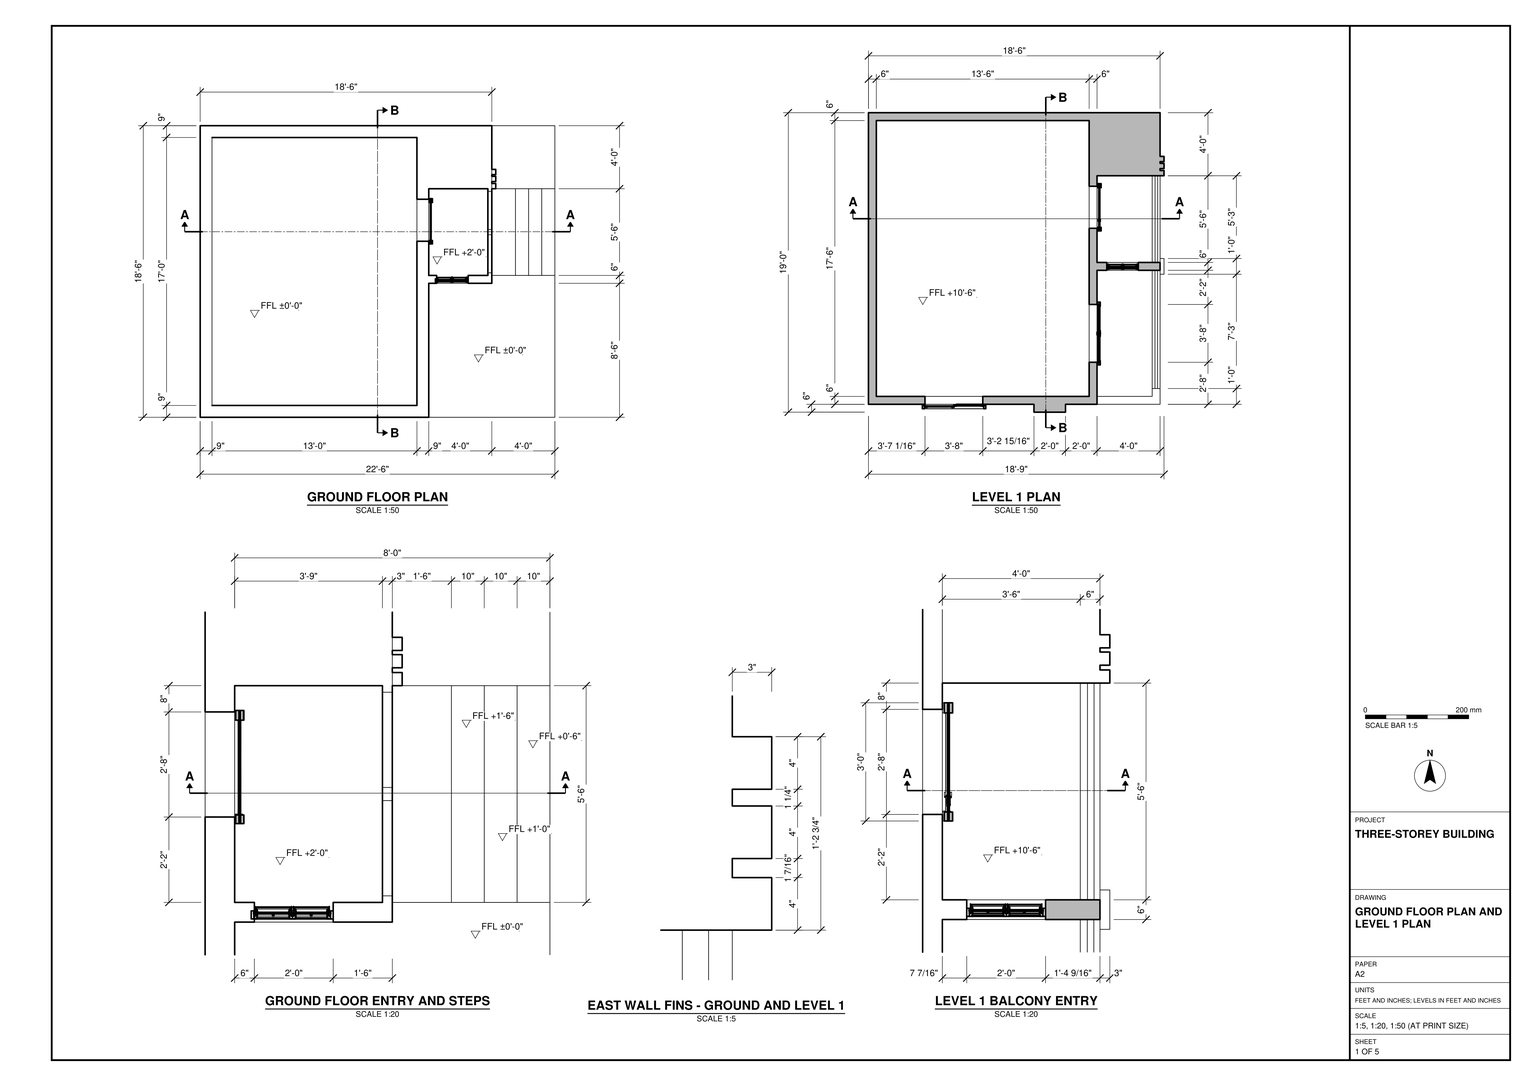
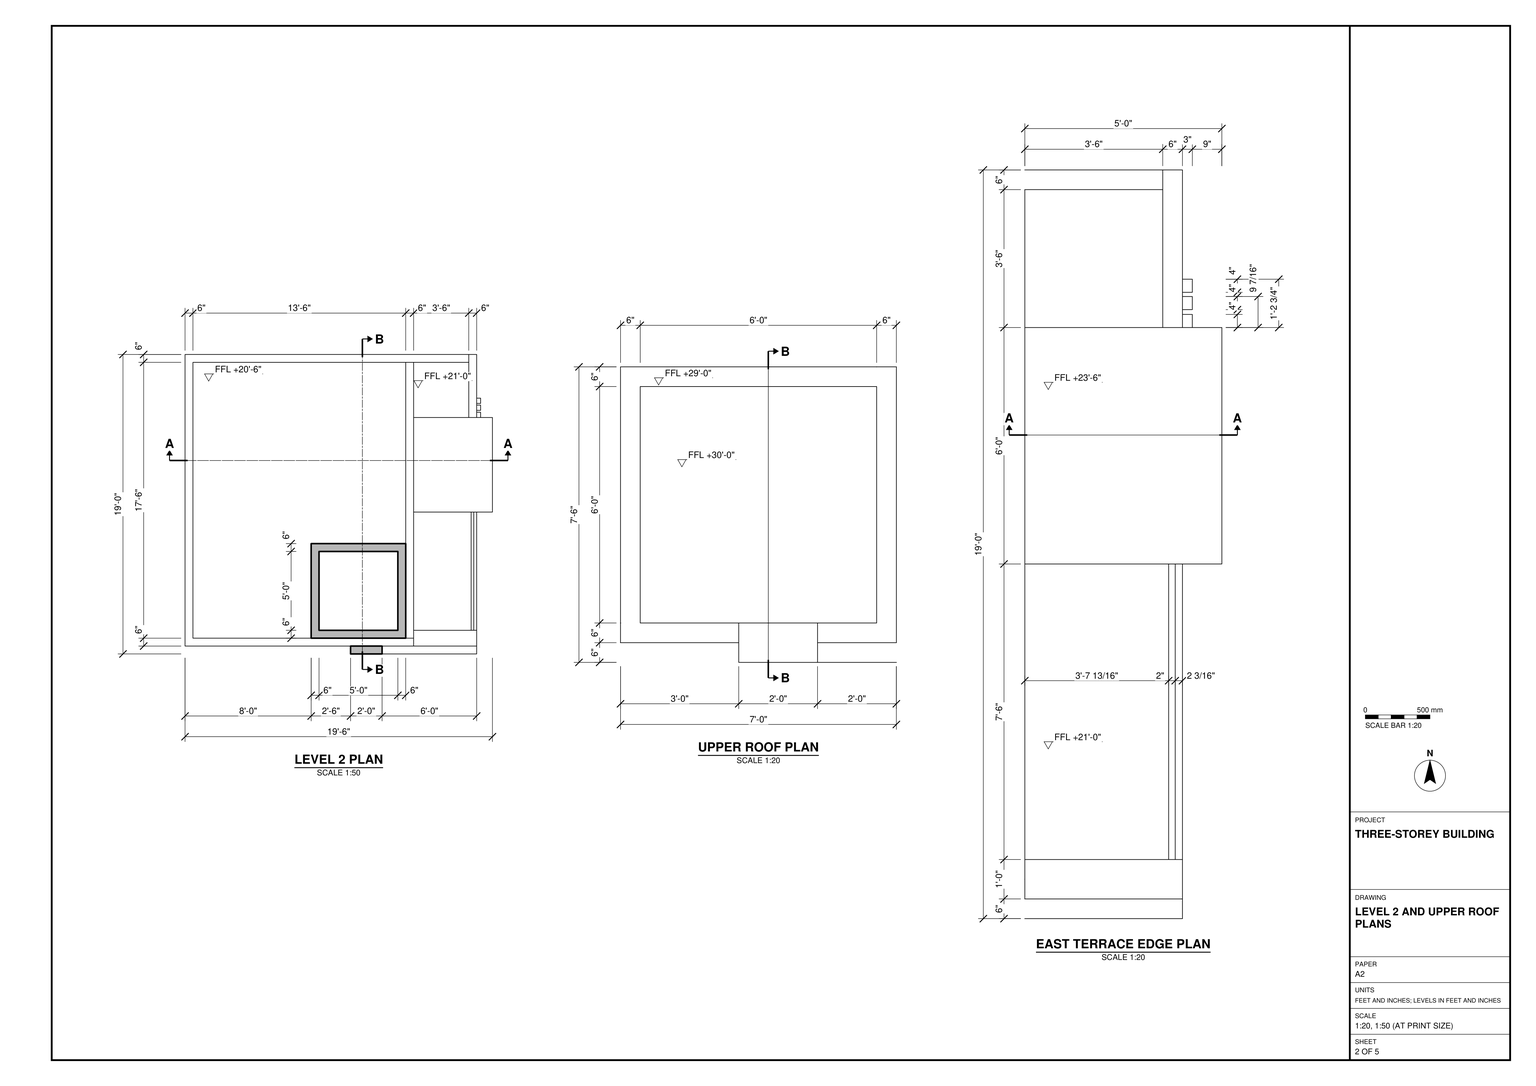
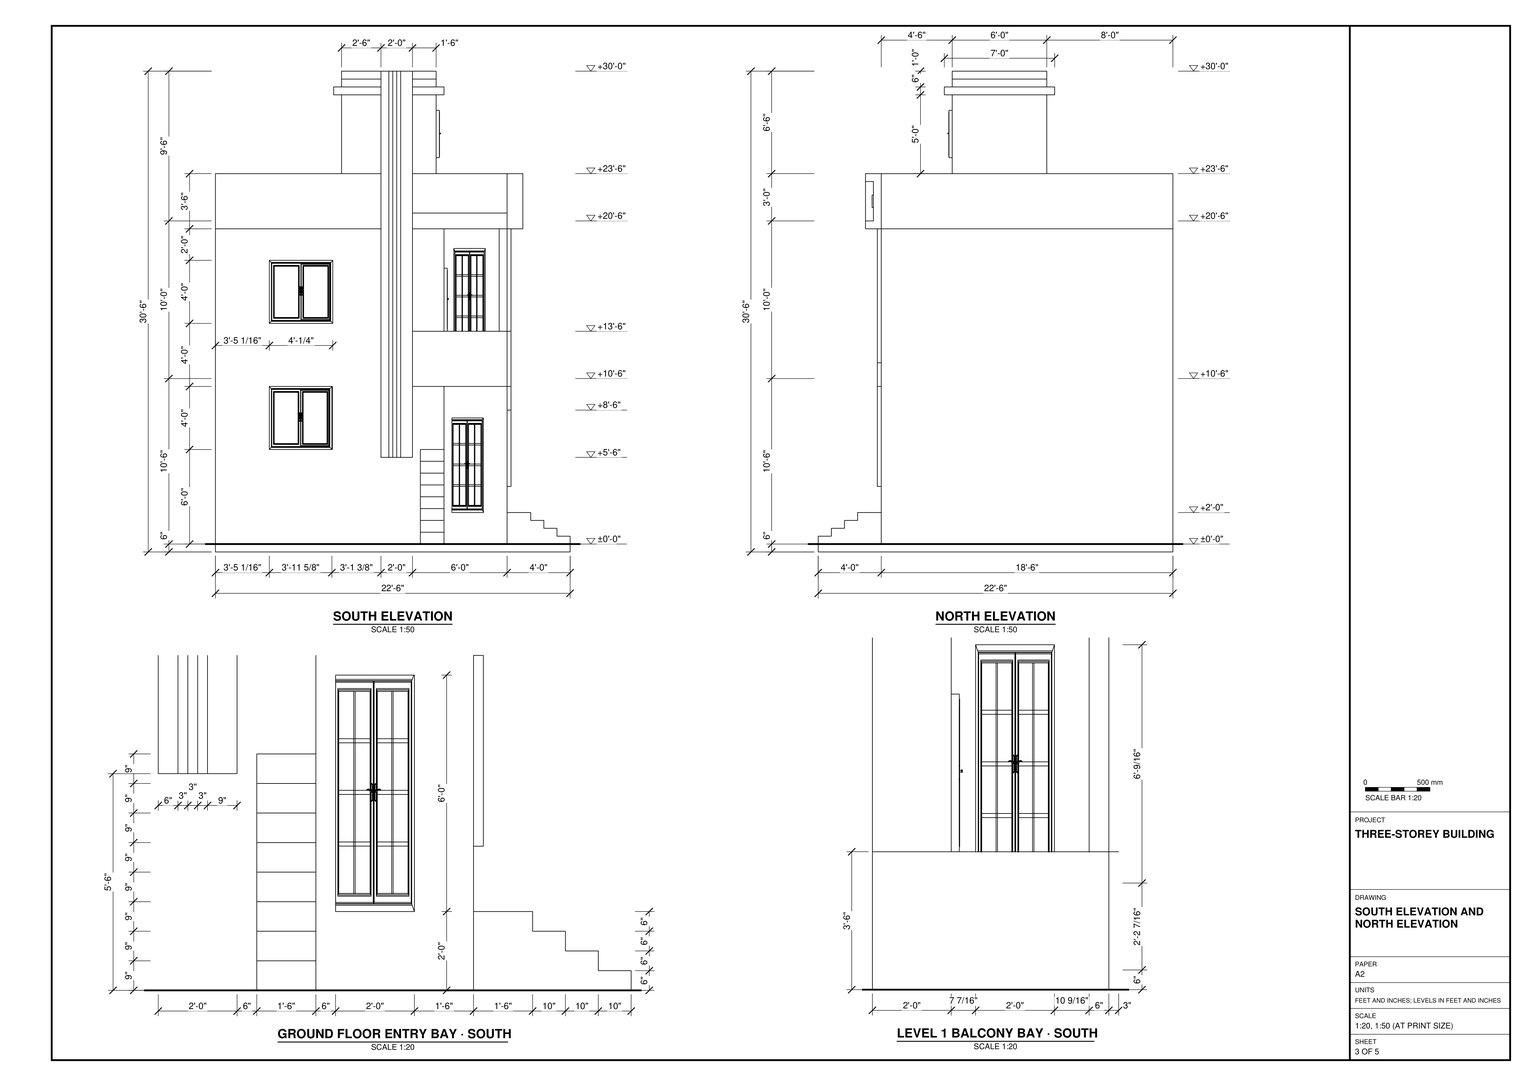
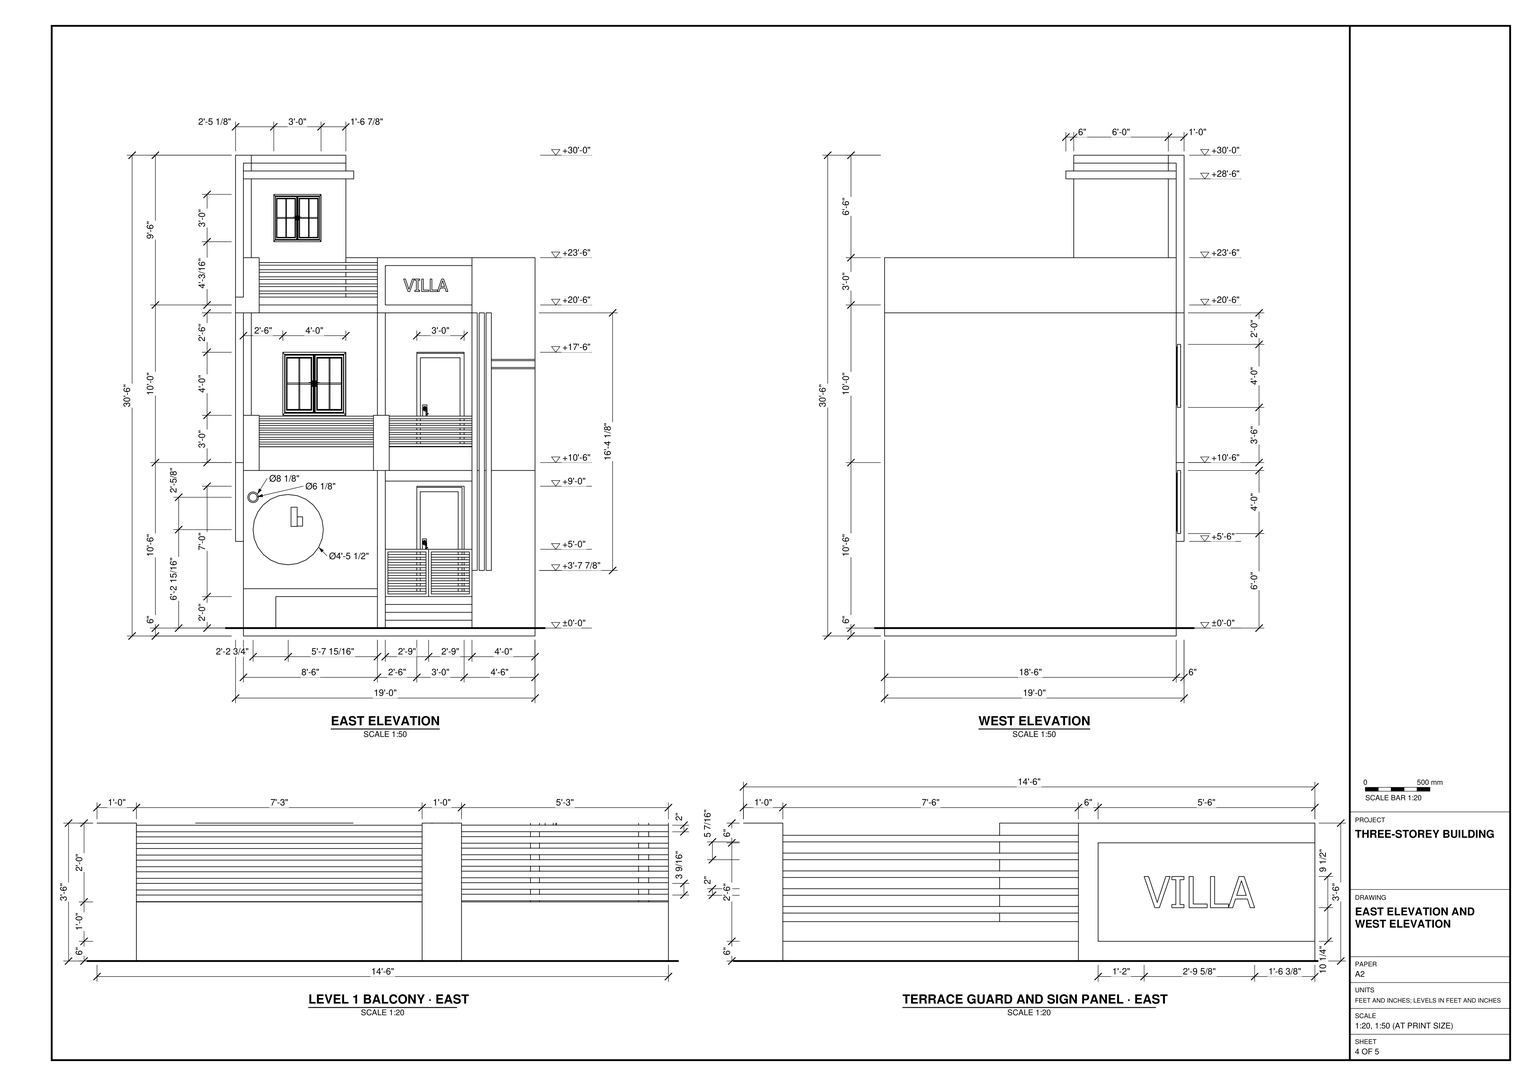
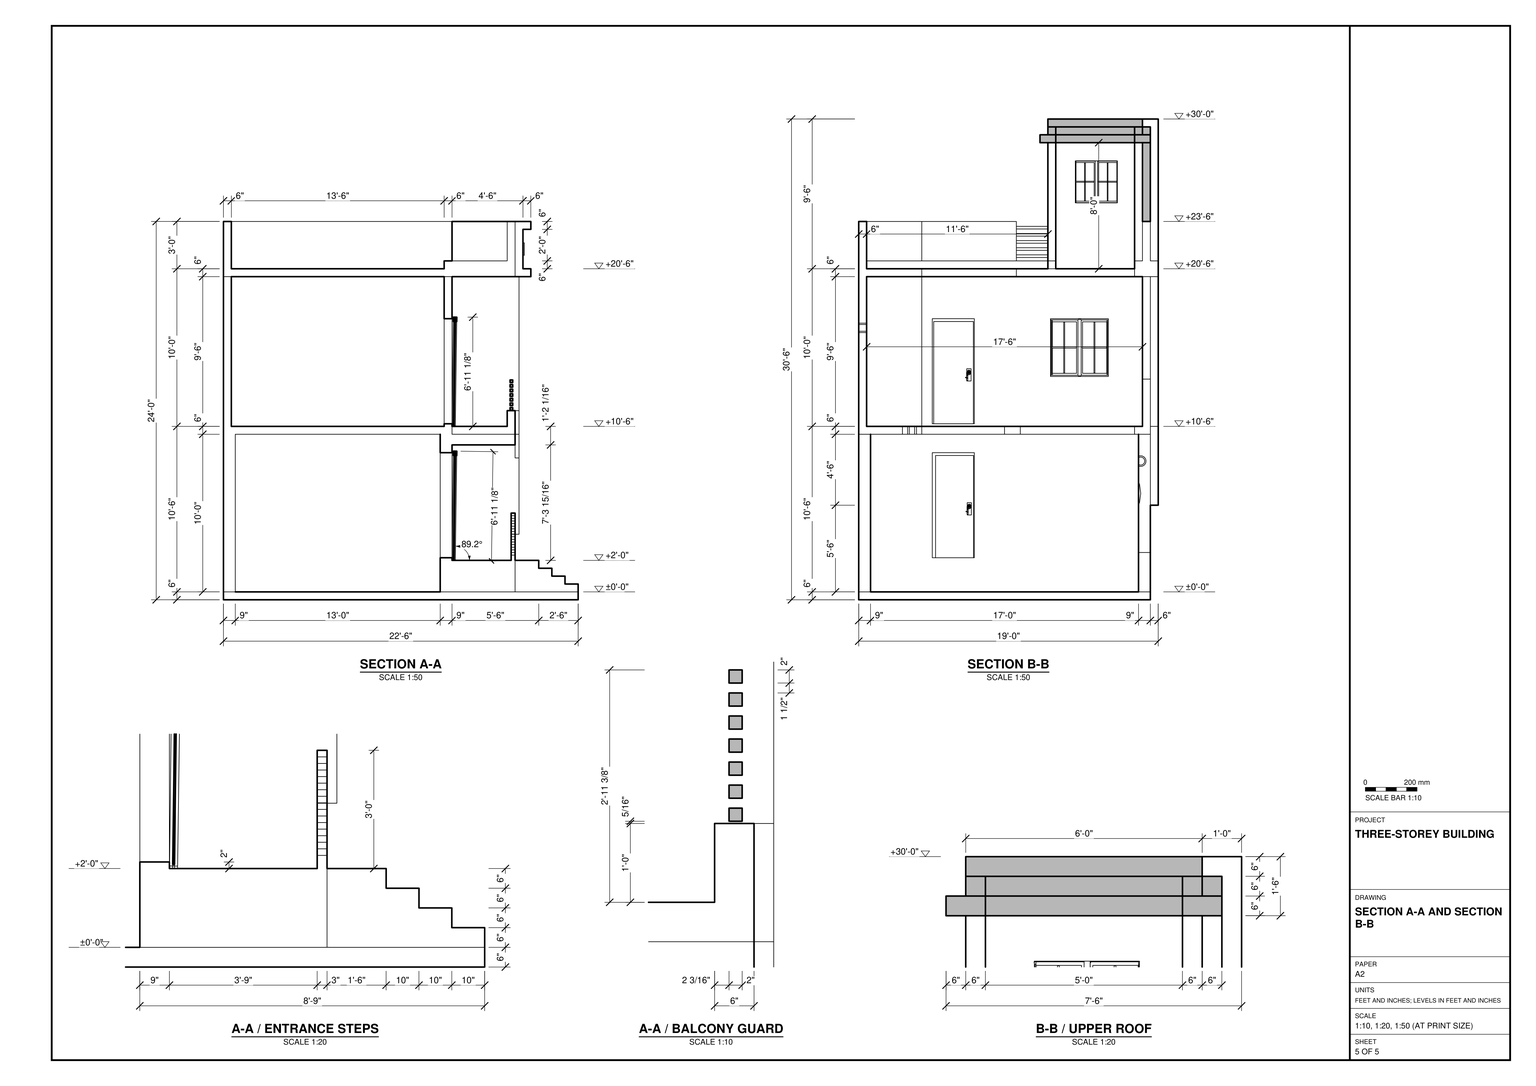
Model the three-storey building in SketchUp using task_files/diagram_01.pdf. Work in feet and inches. The overall model measures 22'-6" east to west, 19'-0" north to south and 30'-6" from the underside of the base slab to the highest roof surface. Set the ground floor at ±0'-0", Level 1 at +10'-6" and Level 2 at +20'-6".

Build the base and floor slabs to the plan outlines. Use the drawn wall thicknesses, including 9" for the main ground-floor walls and 6" for the main Level 1 walls. On the east side, form the exterior steps up to the +2'-0" entry landing and model the balcony above. Fit the doors and framed window units in their drawn positions. Use the south elevation to align the paired windows on the two lower floors and to locate the tall, narrow glazed openings in the entry and balcony bays. Include the projecting east wall fins and the vertical ribbed strip on the south face.

Form the open Level 2 terrace with its parapets, projecting east edge and small rooftop enclosure with an overhanging flat roof. Keep walls, slabs, roof elements and any individual furniture or joinery pieces in separate groups or components. Use components for repeated parts. Any decor or loose items may be suitable library components. Save one SketchUp model as output_files/three_storey_building_east_balcony_and_roof_terrace.skp.

# SketchUp Ruby script. Lengths in inches.
U = 1.inch
M = Sketchup.active_model
def pt(a) = Geom::Point3d.new(a.map { |v| v * U })
def face(e, loops, mat)
  f = e.add_face(loops[0].map { |a| pt(a) })
  loops[1..].each { |l| e.add_face(l.map { |a| pt(a) }).erase! }
  f.material = f.back_material = mat if mat
  f
end
# faces: each face lists its corners as indices into pts; further lists are holes
def faces(e, pts, list, mat = nil) = list.each { |f| face(e, (f[0].is_a?(Array) ? f : [f]).map { |l| l.map { |i| pts[i] } }, mat) }
# xy, xz, yz: faces in a plane at the given z, y or x. An outline is a flat list of corners, or four numbers for a rectangle; further outlines are holes
def ring(l) = l.size == 4 ? [[l[0], l[1]], [l[2], l[1]], [l[2], l[3]], [l[0], l[3]]] : l.each_slice(2).to_a
def flat(e, list, mat, &to3) = list.each { |f| face(e, (f[0].is_a?(Array) ? f : [f]).map { |l| ring(l).map { |u, v| to3.(u, v) } }, mat) }
def xy(e, z, list, mat = nil) = flat(e, list, mat) { |x, y| [x, y, z] }
def xz(e, y, list, mat = nil) = flat(e, list, mat) { |x, z| [x, y, z] }
def yz(e, x, list, mat = nil) = flat(e, list, mat) { |y, z| [x, y, z] }
def lines(e, pts, list) = list.each { |a, b| e.add_line(pt(pts[a]), pt(pts[b])) }
# prism: a flat outline (further loops are holes) pulled along v
def prism(e, loops, v, mat = nil)
  f = face(e, loops, mat); d = Geom::Vector3d.new(v.map { |x| x * U })
  f.pushpull(f.normal.samedirection?(d) ? d.length : -d.length)
end
def box(e, o, s, mat = nil) = prism(e, [[o, [o[0] + s[0], o[1], o[2]], [o[0] + s[0], o[1] + s[1], o[2]], [o[0], o[1] + s[1], o[2]]]], [0, 0, s[2]], mat)
def at(x, y, z, deg = 0) = Geom::Transformation.translation(pt([x, y, z])) * Geom::Transformation.rotation(ORIGIN, Z_AXIS, deg.degrees)
def axes(o, x, y, z) = Geom::Transformation.new([*x, 0, *y, 0, *z, 0, *pt(o).to_a, 1])
def part(name) = M.definitions.add(name)
# library, detail: a bought-in or finely detailed component or shape, given as its bounding box
def library(name, o, s) = part(name).tap { |d| box(d.entities, o, s) }
def detail(e, o, s) = box(e.add_group.entities, o, s)
def put(e, d, t, mat = nil) = e.add_instance(d, t).tap { |i| i.material = mat if mat }
def group(e, t, mat = nil) = e.add_group.tap { |g| g.transformation = t; g.material = mat if mat }.entities
root = M.entities
M.materials.add("C05_Golden_Blaze").color = [255, 123, 0]
M.materials.add("Carpet_04_1K").color = [43, 65, 85]
M.materials.add("D05_Goldenrod_Hue").color = [255, 191, 0]
c1 = library("porta+4",[0.2,-5.42,1.33],[46.55,4.72,83.21])
c2 = part("VILLA")
prism(c2.entities,[[[7.85,9.51,0],[4.58,0,0],[3.22,0,0],[-0.05,9.51,0],[1.3,9.51,0],[3.93,1.62,0],[6.5625,9.51,0]]],[0,0,1])
prism(c2.entities,[[[12.09,0,0],[8.4,0,0],[8.4,0.97,0],[9.61,0.97,0],[9.61,8.54,0],[8.4,8.54,0],[8.4,9.51,0],[12.09,9.51,0],[12.09,8.54,0],[10.875,8.54,0],[10.875,0.97,0],[12.09,0.97,0]]],[0,0,1])
prism(c2.entities,[[[19.16,0,0],[13.65,0,0],[13.65,9.51,0],[14.91,9.51,0],[14.91,1.125,0],[19.16,1.125,0]]],[0,0,1])
xy(c2.entities,0,[[20.15,0,20.15,9.51,21.42,9.51,21.42,1.125,25.66,1.125,25.66,0],[[25.63,0,28.84,9.51,30.4,9.51,33.6,0,32.27,0,31.4,2.66,27.77,2.66,26.91,0],[28.12,3.74,31.05,3.74,29.58,8.22]]])
xy(c2.entities,1,[[20.15,0,25.63,0,25.66,0.09,25.66,1.125,21.42,1.125,21.42,9.51,20.15,9.51],[25.63,0,25.66,0,25.66,0.09],[[25.66,0,26.91,0,27.77,2.66,31.4,2.66,32.27,0,33.6,0,30.4,9.51,28.84,9.51,25.66,0.09],[28.12,3.74,29.58,8.22,31.05,3.74]]])
xz(c2.entities,0,[[20.15,0,25.63,1],[25.63,0,25.66,1],[25.66,0,26.91,1],[32.27,0,33.6,1]])
xz(c2.entities,1.125,[[21.42,0,25.66,1]])
xz(c2.entities,2.66,[[27.77,0,31.4,1]])
xz(c2.entities,3.74,[[28.12,0,31.05,1]])
xz(c2.entities,9.51,[[20.15,0,21.42,1],[28.84,0,30.4,1]])
yz(c2.entities,20.15,[[0,0,9.51,1]])
yz(c2.entities,21.42,[[1.125,0,9.51,1]])
yz(c2.entities,25.66,[[0,0,1.125,1]])
p = [[28.84,9.51,0],[25.63,0,0],[25.63,0,1],[25.66,0.09,1],[28.84,9.51,1],[26.91,0,0],
  [27.77,2.66,0],[27.77,2.66,1],[26.91,0,1],[33.6,0,0],[30.4,9.51,0],[30.4,9.51,1],
  [33.6,0,1],[31.4,2.66,0],[32.27,0,0],[32.27,0,1],[31.4,2.66,1],[28.12,3.74,0],
  [29.58,8.22,0],[29.58,8.22,1],[28.12,3.74,1],[31.05,3.74,0],[31.05,3.74,1]]
faces(c2.entities,p,[[0,1,2,3,4],[5,6,7,8],[9,10,11,12],[13,14,15,16],[17,18,19,20],[18,21,22,19]])
c3 = library("mesh-162",[-1607.75,-1245.64,-53.98],[1739.16,1702.88,120.91])
c4 = part("Group9")
put(c4.entities,c3,at(0,0,0))
c5 = library("mesh-163",[-551.08,-704.17,-20.03],[1929.24,1401.85,86.96])
c6 = part("Group11")
put(c6.entities,c5,at(0,0,0))
c7 = library("mesh-166",[-1553.69,-2604.3125,-42.18],[1702.88,1401.6,88.28])
c8 = part("Group17")
put(c8.entities,c7,at(294.66,859.51,3.5))
xy(root,-6,[[0,6,270,228]])
xy(root,0,[[174,6,270,6,270,114,222,114,222,108,174,108],[9,15,165,219],[222,180,270,228]])
xy(root,6,[[260,114,270,180]])
xy(root,12,[[250,114,260,180]])
xy(root,18,[[240,114,250,180]])
xy(root,24,[[180,108,204,108,204,114,219,114,219,180,174,180,174,114,180,114],[222,114,240,180]])
xy(root,26,[[165,140,174,172]])
xy(root,28,[[219,116,222,145],[219,149,222,178]],"C05_Golden_Blaze")
xy(root,30,[[219,116,222,145],[219,149,222,178]])
xy(root,32,[[219,116,222,145],[219,149,222,178]],"C05_Golden_Blaze")
xy(root,34,[[219,116,222,145],[219,149,222,178]])
xy(root,36,[[219,116,222,145],[219,149,222,178]],"C05_Golden_Blaze")
xy(root,38,[[219,116,222,145],[219,149,222,178]])
xy(root,40,[[219,116,222,145],[219,149,222,178]],"C05_Golden_Blaze")
xy(root,42,[[219,116,222,145],[219,149,222,178]])
xy(root,43.89,[[222,180,225,184],[222,185.45,225,189.45],[222,190.73,225,194.73]],"C05_Golden_Blaze")
xy(root,44,[[219,116,222,145]],"C05_Golden_Blaze")
xy(root,46,[[219,116,222,145],[219,149,222,178]])
xy(root,48,[[219,116,222,145],[219,149,222,178]],"C05_Golden_Blaze")
xy(root,50,[[219,116,222,145],[219,149,222,178]])
xy(root,52,[[219,116,222,145],[219,149,222,178]],"C05_Golden_Blaze")
xy(root,54,[[219,116,222,145],[219,149,222,178]])
xy(root,56,[[219,116,222,145],[219,149,222,178]],"C05_Golden_Blaze")
xy(root,58,[[219,116,222,145],[219,149,222,178]])
xy(root,60,[[219,114,222,180]],"C05_Golden_Blaze")
xy(root,66,[[126,0,147.88,6],[147.88,0,150,6]],"Carpet_04_1K")
xy(root,74,[[43.04,6,87.04,12]])
xy(root,96,[[180,108,204,114]])
xy(root,106,[[165,140,174,172]])
xy(root,111.91,[[174,114,222,180]])
xy(root,118,[[43.04,6,87.04,12]])
xy(root,120,[[174,6,222,108]])
xy(root,120,[[222,105,225,117]],"Carpet_04_1K")
xy(root,126,[[6,12,168,222],[174,12,216,108],[174,114,216,180]])
xy(root,128,[[168,140,174,172]])
xy(root,138,[[216,18,222,108],[216,114,222,180]])
xy(root,138.09,[[218.13,18,220.13,108]])
xy(root,138.34,[[218.2,114,220.2,180]])
xy(root,140.09,[[218.13,18,220.13,108]])
xy(root,140.34,[[218.2,114,220.2,180]])
xy(root,141.63,[[218.13,18,220.13,108]])
xy(root,141.85,[[218.2,114,220.2,180]])
xy(root,143.63,[[218.13,18,220.13,108]])
xy(root,143.85,[[218.2,114,220.2,180]])
xy(root,145.18,[[218.13,18,220.13,108]])
xy(root,145.35,[[218.2,114,220.2,180]])
xy(root,147.18,[[218.13,18,220.13,108]])
xy(root,147.35,[[218.2,114,220.2,180]])
xy(root,148.72,[[218.13,18,220.13,108]])
xy(root,148.86,[[218.2,114,220.2,180]])
xy(root,150.72,[[218.13,18,220.13,108]])
xy(root,150.86,[[218.2,114,220.2,180]])
xy(root,152.27,[[218.13,18,220.13,108]])
xy(root,152.37,[[218.2,114,220.2,180]])
xy(root,153.04,[[181.43,108,205.43,114]])
xy(root,154.27,[[218.13,18,220.13,108]])
xy(root,154.37,[[218.2,114,220.2,180]])
xy(root,155.81,[[218.13,18,220.13,108]])
xy(root,155.875,[[218.2,114,220.2,180]])
xy(root,157.81,[[218.13,18,220.13,108]])
xy(root,157.875,[[218.2,114,220.2,180]])
xy(root,159.35,[[218.13,18,220.13,108]])
xy(root,159.38,[[218.2,114,220.2,180]])
xy(root,161.35,[[218.13,18,220.13,108]])
xy(root,161.38,[[218.2,114,220.2,180]])
xy(root,162,[[174,6,222,6,222,18,216,18,216,12,174,12]])
xy(root,162,[[222,105,225,117]],"Carpet_04_1K")
xy(root,164,[[168,38,174,82]])
xy(root,170,[[43.04,6,87.04,12]])
xy(root,208,[[168,38,174,82],[168,140,174,172]])
xy(root,214,[[43.04,6,87.04,12]])
xy(root,225.04,[[181.43,108,205.43,114]])
xy(root,240,[[174,0,222,12],[6,12,168,222],[174,12,222,108],[174,114,234,180]])
xy(root,240,[[222,180,225,184],[222,185.45,225,189.45],[222,190.73,225,194.73]],"C05_Golden_Blaze")
xy(root,240,[[150,0,174,6],[222,108,234,114]],"Carpet_04_1K")
xy(root,246,[[6,12,96,12,96,84,168,84,168,222,6,222],[102,18,162,78]])
xy(root,246,[[228,114,234,180]],"Carpet_04_1K")
xy(root,252,[[168,12,174,222],[174,18,222,108],[174,180,216,222]])
xy(root,252,[[150,0,222,6]],"Carpet_04_1K")
xy(root,254.6,[[217.79,18,219.79,108]])
xy(root,256.6,[[217.79,18,219.79,108]])
xy(root,260.02,[[217.79,18,219.79,108]])
xy(root,262.02,[[217.79,18,219.79,108]])
xy(root,265.44,[[217.79,18,219.79,108]])
xy(root,267.44,[[217.79,18,219.79,108]])
xy(root,270.86,[[217.79,18,219.79,108]])
xy(root,272.86,[[217.79,18,219.79,108]])
xy(root,276,[[228,114,234,180]],"Carpet_04_1K")
xy(root,276.28,[[217.79,18,219.79,108]])
xy(root,278.28,[[217.79,18,219.79,108]])
xy(root,282,[[0,6,174,6,174,12,6,12,6,222,216,222,216,228,0,228],[174,6,222,18]])
xy(root,282,[[174,108,234,180],[216,180,222,228]],"Carpet_04_1K")
xy(root,296.17,[[162,31.12,168,63.12]])
xy(root,328.17,[[162,31.12,168,63.12]])
xy(root,342,[[[90,6,174,90],[96,12,168,84]],[96,12,168,84]])
xy(root,348,[[[90,6,174,90],[96,12,168,84]],[96,12,168,84]])
xy(root,354,[[126,6,150,12],[96,12,168,18],[96,18,102,84],[102,18,162,78],[162,18,168,84],
  [102,78,162,84]])
xy(root,360,[[126,0,150,12],[96,12,168,84]],"Carpet_04_1K")
xz(root,0,[[132,66,135,360],[138,66,141,360]])
xz(root,0,[[126,66,132,360],[135,66,138,360],[141,66,150,360],[150,240,222,252]],"Carpet_04_1K")
xz(root,6,[[0,-6,270,0],[[0,0,156,0,156,72,174,72,174,120,150,120,150,66,126,66,126,240,0,240],[41.04,168,89.04,216],[41.04,72,89.04,120]],[[41.04,72,89.04,120],[43.04,74,87.04,118]],[150,120,222,162],[150,162,174,240],
  [[41.04,168,89.04,216],[43.04,170,87.04,214]],[0,240,126,282],[150,252,222,282],[126,282,150,342],[90,342,126,348],
  [126,342,150,348],[150,342,174,348],[126,348,150,354]])
xz(root,6,[[156,0,174,9],[156,9,174,18],[156,18,174,27],[156,27,174,36],[156,36,174,45],
  [156,45,174,54],[156,54,174,63],[156,63,174,72]],"Carpet_04_1K")
xz(root,12,[[43.04,74,87.04,118],[[6,126,168,240],[43.04,170,87.04,214]],[174,126,216,162],[6,246,96,282],[168,252,174,282],
  [96,282,168,342],[96,348,168,354],[126,354,150,360]])
xz(root,12,[[96,354,126,360],[150,354,168,360]],"Carpet_04_1K")
xz(root,15,[[9,0,165,120]])
xz(root,18,[[[216,138,222,162],[218.13,159.35,220.13,161.35],[218.13,155.81,220.13,157.81],[218.13,152.27,220.13,154.27],[218.13,148.72,220.13,150.72],[218.13,145.18,220.13,147.18],[218.13,141.63,220.13,143.63],[218.13,138.09,220.13,140.09]],[102,246,162,354],[[174,252,222,282],[217.79,276.28,219.79,278.28],[217.79,270.86,219.79,272.86],[217.79,265.44,219.79,267.44],[217.79,260.02,219.79,262.02],[217.79,254.6,219.79,256.6]]])
xz(root,31.12,[[162,296.17,168,328.17]])
xz(root,38,[[168,164,174,208]])
xz(root,63.12,[[162,296.17,168,328.17]])
xz(root,78,[[102,246,162,354]])
xz(root,82,[[168,164,174,208]])
xz(root,84,[[96,246,168,342],[96,348,168,354]])
xz(root,84,[[96,354,168,360]],"Carpet_04_1K")
xz(root,90,[[90,342,174,348]])
xz(root,105,[[222,120,225,162]],"Carpet_04_1K")
xz(root,108,[[[174,0,222,120],[180,24,204,96]],[[174,126,216,240],[181.43,153.04,205.43,225.04]],[[216,138,222,240],[218.13,159.35,220.13,161.35],[218.13,155.81,220.13,157.81],[218.13,152.27,220.13,154.27],[218.13,148.72,220.13,150.72],[218.13,145.18,220.13,147.18],[218.13,141.63,220.13,143.63],[218.13,138.09,220.13,140.09]]])
xz(root,108,[[[222,240,234,240,234,282,174,282,174,252,222,252],[217.79,276.28,219.79,278.28],[217.79,270.86,219.79,272.86],[217.79,265.44,219.79,267.44],[217.79,260.02,219.79,262.02],[217.79,254.6,219.79,256.6]]],"Carpet_04_1K")
xz(root,114,[[222,0,270,0,270,6,260,6,260,12,250,12,250,18,240,18,240,24,222,24],[174,24,174,111.91,222,111.91,222,60,219,60,219,24,204,24,204,96,180,96,180,24],[[174,126,216,240],[181.43,153.04,205.43,225.04]],[[216,138,222,240],[218.2,138.34,220.2,140.34],[218.2,141.85,220.2,143.85],[218.2,145.35,220.2,147.35],[218.2,148.86,220.2,150.86],[218.2,152.37,220.2,154.37],[218.2,155.875,220.2,157.875],[218.2,159.38,220.2,161.38]]])
xz(root,114,[[228,246,234,276]],"Carpet_04_1K")
xz(root,116,[[219,28,222,30],[219,32,222,34],[219,36,222,38],[219,40,222,42],[219,44,222,46],
  [219,48,222,50],[219,52,222,54],[219,56,222,58]])
xz(root,117,[[222,120,225,162]],"Carpet_04_1K")
xz(root,140,[[165,26,174,106],[168,128,174,208]])
xz(root,145,[[219,28,222,30],[219,32,222,34],[219,36,222,38],[219,40,222,42],[219,44,222,46],
  [219,48,222,50],[219,52,222,54],[219,56,222,58]])
xz(root,149,[[219,28,222,30],[219,32,222,34],[219,36,222,38],[219,40,222,42],[219,44,222,46],
  [219,48,222,50],[219,52,222,54],[219,56,222,58]])
xz(root,172,[[165,26,174,106],[168,128,174,208]])
xz(root,178,[[219,28,222,30],[219,32,222,34],[219,36,222,38],[219,40,222,42],[219,43.89,222,46],
  [219,48,222,50],[219,52,222,54],[219,56,222,58]])
xz(root,180,[[222,0,222,24,240,24,240,18,250,18,250,12,260,12,260,6,270,6,270,0],[174,24,219,24,219,60,222,60,222,43.89,225,43.89,225,102,222,102,222,111.91,174,111.91],[174,120,222,120,222,138,216,138,216,126,174,126],[[174,126,216,126,216,138,225,138,225,240,174,240],[218.2,159.38,220.2,161.38],[218.2,155.875,220.2,157.875],[218.2,152.37,220.2,154.37],[218.2,148.86,220.2,150.86],[218.2,145.35,220.2,147.35],[218.2,141.85,220.2,143.85],[218.2,138.34,220.2,140.34]]])
xz(root,180,[[222,102,225,120],[222,120,225,138]],"C05_Golden_Blaze")
xz(root,180,[[222,240,222,282,234,282,234,276,228,276,228,246,234,246,234,240],[174,252,216,282]],"Carpet_04_1K")
xz(root,184,[[222,43.89,225,120],[222,120,225,138],[222,138,225,240]],"C05_Golden_Blaze")
xz(root,185.45,[[222,43.89,225,102],[222,102,225,120],[222,120,225,138],[222,138,225,240]],"C05_Golden_Blaze")
xz(root,189.45,[[222,43.89,225,120],[222,120,225,138],[222,138,225,240]],"C05_Golden_Blaze")
xz(root,190.73,[[222,43.89,225,102],[222,102,225,120],[222,120,225,138],[222,138,225,240]],"C05_Golden_Blaze")
xz(root,194.73,[[222,43.89,225,120],[222,120,225,138],[222,138,225,240]],"C05_Golden_Blaze")
xz(root,219,[[9,0,165,120]])
xz(root,222,[[6,126,168,240],[6,246,168,246,168,252,216,252,216,282,6,282]])
xz(root,228,[[0,-6,270,0],[0,0,222,240],[0,240,222,282]])
yz(root,0,[[6,-6,228,0],[6,0,228,240],[6,240,228,282]])
yz(root,6,[[12,126,222,240],[12,246,222,282]])
yz(root,43.04,[[6,74,12,118],[6,170,12,214]])
yz(root,87.04,[[6,74,12,118],[6,170,12,214]])
yz(root,90,[[6,342,90,348]])
yz(root,96,[[12,246,84,342],[12,348,84,354]])
yz(root,96,[[12,354,84,360]],"Carpet_04_1K")
yz(root,102,[[18,246,78,354]])
yz(root,126,[[0,66,6,126],[0,126,6,240],[0,240,0,360,12,360,12,354,6,354,6,240]],"Carpet_04_1K")
yz(root,150,[[0,66,6,126],[0,126,6,240],[0,252,6,252,6,354,12,354,12,360,0,360]],"Carpet_04_1K")
yz(root,162,[[[18,246,78,354],[31.12,296.17,63.12,328.17]]])
yz(root,165,[[[15,0,219,120],[140,26,172,106]]])
yz(root,168,[[[12,126,180,240],[140,128,172,208],[38,164,82,208]],[180,126,222,240],[84,246,222,252],[[12,252,84,342],[29.12,294.17,65.12,330.17]],[[29.12,294.17,65.12,330.17],[31.12,296.17,63.12,328.17]],
  [12,348,84,354]])
yz(root,168,[[12,354,84,360]],"Carpet_04_1K")
yz(root,174,[[30.67,0,108,24],[114,24,138,24,138,108,174,108,174,24,180,24,180,111.91,114,111.91],[[138,24,174,108],[140,26,172,106]],[[6,30,108,120],[40.09,48.2,33.16,49.12,26.71,51.79,21.17,56.04,16.91,61.59,14.24,68.04,13.33,74.97,14.24,81.9,16.91,88.35,21.17,93.89,26.71,98.15,33.16,100.82,40.09,101.73,47.02,100.82,53.47,98.15,59.02,93.89,63.27,88.35,65.94,81.9,66.86,74.97,65.94,68.04,63.27,61.59,59.02,56.04,53.47,51.79,47.02,49.12],[13.83,95.5625,12.77,95.58,11.76,95.87,10.85,96.41,10.11,97.17,9.59,98.1,9.34,99.12,9.35,100.18,9.64,101.2,10.1875,102.11,10.95,102.85,11.87,103.36,12.9,103.62,13.96,103.6,14.97,103.3125,15.88,102.77,16.62,102.01,17.14,101.08,17.39,100.06,17.38,99,17.09,97.98,16.54,97.07,15.78,96.34,14.86,95.82]],[[13.83,95.5625,14.86,95.82,15.78,96.34,16.54,97.07,17.09,97.98,17.38,99,17.39,100.06,17.14,101.08,16.62,102.01,15.88,102.77,14.97,103.3125,13.96,103.6,12.9,103.62,11.87,103.36,10.95,102.85,10.1875,102.11,9.64,101.2,9.35,100.18,9.34,99.12,9.59,98.1,10.11,97.17,10.85,96.41,11.76,95.87,12.77,95.58],[13.72,96.55,12.92,96.57,12.15,96.79,11.47,97.19,10.91,97.77,10.52,98.46,10.33,99.24,10.34,100.04,10.56,100.8,10.97,101.49,11.54,102.04,12.24,102.43,13.01,102.625,13.81,102.61,14.58,102.4,15.26,101.99,15.82,101.41,16.21,100.72,16.4,99.94,16.39,99.14,16.17,98.38,15.76,97.69,15.1875,97.14,14.49,96.75]],
  [13.72,96.55,14.49,96.75,15.1875,97.14,15.76,97.69,16.17,98.38,16.39,99.14,16.4,99.94,16.21,100.72,15.82,101.41,15.26,101.99,14.58,102.4,13.81,102.61,13.01,102.625,12.24,102.43,11.54,102.04,10.97,101.49,10.56,100.8,10.34,100.04,10.33,99.24,10.52,98.46,10.91,97.77,11.47,97.19,12.15,96.79,12.92,96.57],[[12,126,108,240],[36,162,84,210]],[114,126,138,126,138,210,174,210,174,126,180,126,180,240,114,240],[[138,126,174,210],[140,128,172,208]],[6,162,12,240],
  [[36,162,84,210],[38,164,82,208]],[12,252,18,282],[6,342,90,348]])
yz(root,174,[[6,0,30.67,0,30.67,24,108,24,108,30,6,30],[[40.09,48.2,47.02,49.12,53.47,51.79,59.02,56.04,63.27,61.59,65.94,68.04,66.86,74.97,65.94,81.9,63.27,88.35,59.02,93.89,53.47,98.15,47.02,100.82,40.09,101.73,33.16,100.82,26.71,98.15,21.17,93.89,16.91,88.35,14.24,81.9,13.33,74.97,14.24,68.04,16.91,61.59,21.17,56.04,26.71,51.79,33.16,49.12],[42.26,77.4,42.26,92.04,46.93,92.04,46.93,84.72,51.08,84.72,51.08,77.67,46.93,77.67,46.93,77.4]],[108,252,180,282]],"Carpet_04_1K")
yz(root,174,[[42.26,77.4,46.93,92.04],[46.93,77.67,51.08,84.72]],"D05_Goldenrod_Hue")
yz(root,180,[[108,24,114,96]])
yz(root,181.43,[[108,153.04,114,225.04]])
yz(root,204,[[108,24,114,96]])
yz(root,205.43,[[108,153.04,114,225.04]])
yz(root,216,[[12,126,108,138],[114,126,180,138],[12,138,18,162],[180,252,222,282]])
yz(root,217.79,[[18,254.6,108,256.6],[18,260.02,108,262.02],[18,265.44,108,267.44],[18,270.86,108,272.86],[18,276.28,108,278.28]])
yz(root,218.13,[[18,138.09,108,140.09],[18,141.63,108,143.63],[18,145.18,108,147.18],[18,148.72,108,150.72],[18,152.27,108,154.27],
  [18,155.81,108,157.81],[18,159.35,108,161.35]])
yz(root,218.2,[[114,138.34,180,140.34],[114,141.85,180,143.85],[114,145.35,180,147.35],[114,148.86,180,150.86],[114,152.37,180,154.37],
  [114,155.875,180,157.875],[114,159.38,180,161.38]])
yz(root,219,[[[114,24,180,60],[178,43.89,178,46,149,46,149,44],[116,52,145,54],[116,48,145,50],[116,44,145,46],[116,40,145,42],[116,36,145,38],[116,32,145,34],[149,52,178,54],[149,48,178,50],[149,40,178,42],[149,36,178,38],[149,32,178,34],[149,56,178,58],[116,56,145,58],[116,28,145,30],[149,28,178,30]]])
yz(root,219.79,[[18,254.6,108,256.6],[18,260.02,108,262.02],[18,265.44,108,267.44],[18,270.86,108,272.86],[18,276.28,108,278.28]])
yz(root,220.13,[[18,138.09,108,140.09],[18,141.63,108,143.63],[18,145.18,108,147.18],[18,148.72,108,150.72],[18,152.27,108,154.27],
  [18,155.81,108,157.81],[18,159.35,108,161.35]])
yz(root,220.2,[[114,138.34,180,140.34],[114,141.85,180,143.85],[114,145.35,180,147.35],[114,148.86,180,150.86],[114,152.37,180,154.37],
  [114,155.875,180,157.875],[114,159.38,180,161.38]])
yz(root,222,[[108,0,114,120],[180,0,228,0,228,120,194.73,120,194.73,43.89,190.73,43.89,190.73,120,189.45,120,189.45,43.89,185.45,43.89,185.45,120,184,120,184,43.89,180,43.89],[114,111.91,180,120],[6,120,18,162],[105,120,117,120,117,138,114,138,114,162,108,162,108,138,105,138],
  [105,138,108,162],[114,138,117,162],[108,162,114,240],[194.73,197.43,228,198.43],[194.73,203.59,228,204.59],
  [0,240,18,240,18,282,6,282,6,252,0,252],[18,246,108,252]])
yz(root,222,[[[114,24,147,60],[116,26,145,58]],[[147,24,180,60],[149,26,178,58]],[116,26,145,28],[149,26,178,28],[116,30,145,32],
  [149,30,178,32],[116,34,145,36],[149,34,178,36],[116,38,145,40],[149,38,178,40],
  [116,42,145,44],[149,42,178,42,178,43.89,149,44],[116,46,145,48],[149,46,178,48],[116,50,145,52],
  [149,50,178,52],[116,54,145,56],[149,54,178,56]],"C05_Golden_Blaze")
yz(root,222,[[18,120,105,138],[117,120,180,138],[184,120,185.45,120,185.45,240,189.45,240,189.45,120,190.73,120,190.73,240,194.73,240,194.73,204.59,228,204.59,228,282,180,282,180,240,184,240],[194.73,120,228,197.43],[194.73,198.43,228,203.59],
  [18,240,108,246]],"Carpet_04_1K")
yz(root,225,[[180,43.89,184,240],[185.45,43.89,189.45,240],[190.73,43.89,194.73,240]],"C05_Golden_Blaze")
yz(root,225,[[105,120,117,162]],"Carpet_04_1K")
yz(root,228,[[114,246,180,276]],"Carpet_04_1K")
yz(root,234,[[108,240,180,240,180,246,114,246,114,276,180,276,180,282,108,282]],"Carpet_04_1K")
yz(root,240,[[114,18,180,24]])
yz(root,250,[[114,12,180,18]])
yz(root,260,[[114,6,180,12]])
yz(root,270,[[6,-6,228,0],[114,0,180,6]])
p = [[222,149,44],[222,178,43.89],[219,178,43.89],[219,149,44],[174,228,120],[174,180,120]]
faces(root,p,[[0,1,2,3]],"C05_Golden_Blaze")
lines(root,p,[[4,5]])
put(root,c1,axes([172.21,137.85,22.66],[0,0.74,0],[-1,0,0],[0,0,1]))
put(root,c1,axes([172.21,137.84,124.66],[0,0.77339,0],[-1,0,0],[0,0,1]))
put(root,c2,axes([228,128.05,256.23],[0,1,0],[0,0,1],[1,0,0]))
put(root,c4,axes([185.74,110.63,91.1],[0,0,0.04173],[-0.01466,0,0],[0,-0.03937,0]))
put(root,c6,axes([174.79,49.65,186.12],[0,0.02476,0],[0,0,0.03425],[0.03937,0,0]))
put(root,c6,axes([168.79,39.35,312.26],[0,0.01857,0],[0,0,0.02569],[0.03937,0,0]))
put(root,c8,axes([76.23,4.48,131.76],[0.02795,0,0],[0,0,0.03425],[0,-0.03937,0]))
put(root,c8,axes([76.73,4.48,227.76],[0.02835,0,0],[0,0,0.03425],[0,-0.03937,0]))
put(root,c4,axes([187.87,110.63,219.5625],[0,0,0.04173],[-0.01409,0,0],[0,-0.03937,0]))
